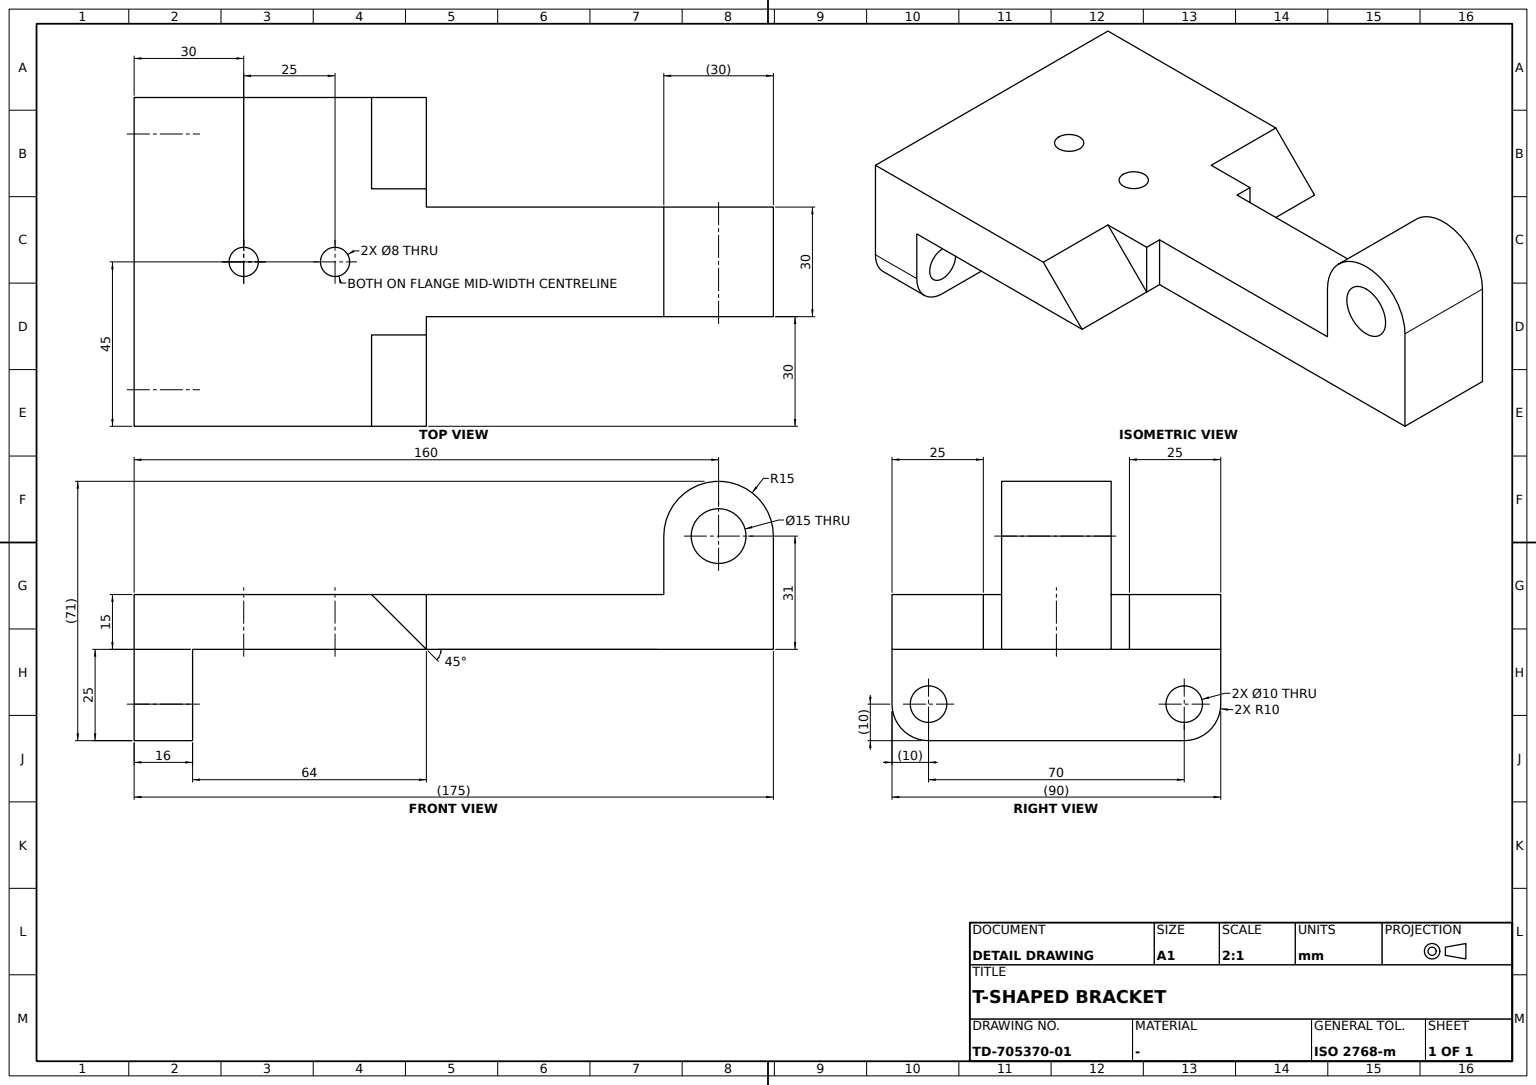
ISO-10303-21;
HEADER;
FILE_DESCRIPTION((''),'2;1');
FILE_NAME('','',(''),(''),'','','');
FILE_SCHEMA(('AUTOMOTIVE_DESIGN'));
ENDSEC;
DATA;
#1=APPLICATION_CONTEXT('');
#2=PRODUCT_CONTEXT('',#1,'mechanical');
#3=PRODUCT('','','',(#2));
#4=PRODUCT_DEFINITION_FORMATION('','',#3);
#5=PRODUCT_DEFINITION_CONTEXT('',#1,'design');
#6=PRODUCT_DEFINITION('','',#4,#5);
#7=PRODUCT_DEFINITION_SHAPE('','',#6);
#8=(LENGTH_UNIT()NAMED_UNIT(*)SI_UNIT(.MILLI.,.METRE.));
#9=(NAMED_UNIT(*)PLANE_ANGLE_UNIT()SI_UNIT($,.RADIAN.));
#10=(NAMED_UNIT(*)SI_UNIT($,.STERADIAN.)SOLID_ANGLE_UNIT());
#11=UNCERTAINTY_MEASURE_WITH_UNIT(LENGTH_MEASURE(0.005),#8,'distance_accuracy_value','');
#12=(GEOMETRIC_REPRESENTATION_CONTEXT(3)GLOBAL_UNCERTAINTY_ASSIGNED_CONTEXT((#11))GLOBAL_UNIT_ASSIGNED_CONTEXT((#8,#9,#10))REPRESENTATION_CONTEXT('',''));
#13=CARTESIAN_POINT('',(160.,-15.,38.5));
#14=VERTEX_POINT('',#13);
#15=CARTESIAN_POINT('',(160.,15.,38.5));
#16=VERTEX_POINT('',#15);
#17=CARTESIAN_POINT('',(160.,75.,38.5));
#18=DIRECTION('',(0.,-1.,0.));
#19=VECTOR('',#18,1000.);
#20=LINE('',#17,#19);
#21=EDGE_CURVE('',#14,#16,#20,.F.);
#22=ORIENTED_EDGE('',*,*,#21,.T.);
#23=CARTESIAN_POINT('',(160.,15.,23.5));
#24=VERTEX_POINT('',#23);
#25=CARTESIAN_POINT('',(160.,15.,31.));
#26=DIRECTION('',(0.,1.,0.));
#27=DIRECTION('',(0.,0.,1.));
#28=AXIS2_PLACEMENT_3D('',#25,#26,#27);
#29=CIRCLE('',#28,7.5);
#30=EDGE_CURVE('',#16,#24,#29,.T.);
#31=ORIENTED_EDGE('',*,*,#30,.T.);
#32=CARTESIAN_POINT('',(160.,-15.,23.5));
#33=VERTEX_POINT('',#32);
#34=CARTESIAN_POINT('',(160.,75.,23.5));
#35=LINE('',#34,#19);
#36=EDGE_CURVE('',#24,#33,#35,.T.);
#37=ORIENTED_EDGE('',*,*,#36,.T.);
#38=CARTESIAN_POINT('',(160.,-15.,31.));
#39=DIRECTION('',(1.,0.,0.));
#40=AXIS2_PLACEMENT_3D('',#38,#18,#39);
#41=CIRCLE('',#40,7.5);
#42=EDGE_CURVE('',#33,#14,#41,.T.);
#43=ORIENTED_EDGE('',*,*,#42,.T.);
#44=EDGE_LOOP('',(#22,#31,#37,#43));
#45=FACE_BOUND('',#44,.T.);
#46=CARTESIAN_POINT('',(160.,75.,31.));
#47=DIRECTION('',(0.,0.,-1.));
#48=AXIS2_PLACEMENT_3D('',#46,#18,#47);
#49=CYLINDRICAL_SURFACE('',#48,7.5);
#50=ADVANCED_FACE('',(#45),#49,.F.);
#51=CARTESIAN_POINT('',(0.,-35.,-10.));
#52=VERTEX_POINT('',#51);
#53=CARTESIAN_POINT('',(16.,-35.,-10.));
#54=VERTEX_POINT('',#53);
#55=DIRECTION('',(-1.,0.,0.));
#56=VECTOR('',#55,1000.);
#57=LINE('',#53,#56);
#58=EDGE_CURVE('',#52,#54,#57,.F.);
#59=ORIENTED_EDGE('',*,*,#58,.T.);
#60=CARTESIAN_POINT('',(16.,-35.,-20.));
#61=VERTEX_POINT('',#60);
#62=CARTESIAN_POINT('',(16.,-35.,-15.));
#63=AXIS2_PLACEMENT_3D('',#62,#39,#26);
#64=CIRCLE('',#63,5.);
#65=EDGE_CURVE('',#54,#61,#64,.T.);
#66=ORIENTED_EDGE('',*,*,#65,.T.);
#67=CARTESIAN_POINT('',(0.,-35.,-20.));
#68=VERTEX_POINT('',#67);
#69=LINE('',#60,#56);
#70=EDGE_CURVE('',#61,#68,#69,.T.);
#71=ORIENTED_EDGE('',*,*,#70,.T.);
#72=CARTESIAN_POINT('',(0.,-35.,-15.));
#73=AXIS2_PLACEMENT_3D('',#72,#39,#26);
#74=CIRCLE('',#73,5.);
#75=EDGE_CURVE('',#52,#68,#74,.T.);
#76=ORIENTED_EDGE('',*,*,#75,.F.);
#77=EDGE_LOOP('',(#59,#66,#71,#76));
#78=FACE_BOUND('',#77,.T.);
#79=AXIS2_PLACEMENT_3D('',#62,#55,#27);
#80=CYLINDRICAL_SURFACE('',#79,5.);
#81=ADVANCED_FACE('',(#78),#80,.F.);
#82=CARTESIAN_POINT('',(59.,0.,15.));
#83=VERTEX_POINT('',#82);
#84=CARTESIAN_POINT('',(51.,0.,15.));
#85=VERTEX_POINT('',#84);
#86=CARTESIAN_POINT('',(55.,0.,15.));
#87=AXIS2_PLACEMENT_3D('',#86,#27,#55);
#88=CIRCLE('',#87,4.);
#89=EDGE_CURVE('',#83,#85,#88,.T.);
#90=ORIENTED_EDGE('',*,*,#89,.T.);
#91=CARTESIAN_POINT('',(51.,0.,0.));
#92=VERTEX_POINT('',#91);
#93=CARTESIAN_POINT('',(51.,0.,90.));
#94=VECTOR('',#47,1000.);
#95=LINE('',#93,#94);
#96=EDGE_CURVE('',#85,#92,#95,.T.);
#97=ORIENTED_EDGE('',*,*,#96,.T.);
#98=CARTESIAN_POINT('',(59.,0.,0.));
#99=VERTEX_POINT('',#98);
#100=CARTESIAN_POINT('',(55.,0.,0.));
#101=AXIS2_PLACEMENT_3D('',#100,#27,#39);
#102=CIRCLE('',#101,4.);
#103=EDGE_CURVE('',#99,#92,#102,.T.);
#104=ORIENTED_EDGE('',*,*,#103,.F.);
#105=CARTESIAN_POINT('',(59.,0.,90.));
#106=LINE('',#105,#94);
#107=EDGE_CURVE('',#99,#83,#106,.F.);
#108=ORIENTED_EDGE('',*,*,#107,.T.);
#109=EDGE_LOOP('',(#90,#97,#104,#108));
#110=FACE_BOUND('',#109,.T.);
#111=CARTESIAN_POINT('',(55.,0.,90.));
#112=AXIS2_PLACEMENT_3D('',#111,#47,#55);
#113=CYLINDRICAL_SURFACE('',#112,4.);
#114=ADVANCED_FACE('',(#110),#113,.F.);
#115=CARTESIAN_POINT('',(0.,45.,15.));
#116=VERTEX_POINT('',#115);
#117=CARTESIAN_POINT('',(0.,45.,-15.));
#118=VERTEX_POINT('',#117);
#119=LINE('',#115,#94);
#120=EDGE_CURVE('',#116,#118,#119,.T.);
#121=ORIENTED_EDGE('',*,*,#120,.T.);
#122=CARTESIAN_POINT('',(0.,35.,-25.));
#123=VERTEX_POINT('',#122);
#124=CARTESIAN_POINT('',(0.,35.,-15.));
#125=AXIS2_PLACEMENT_3D('',#124,#55,#47);
#126=CIRCLE('',#125,10.);
#127=EDGE_CURVE('',#118,#123,#126,.T.);
#128=ORIENTED_EDGE('',*,*,#127,.T.);
#129=CARTESIAN_POINT('',(0.,-35.,-25.));
#130=VERTEX_POINT('',#129);
#131=CARTESIAN_POINT('',(0.,-45.,-25.));
#132=VECTOR('',#26,1000.);
#133=LINE('',#131,#132);
#134=EDGE_CURVE('',#130,#123,#133,.T.);
#135=ORIENTED_EDGE('',*,*,#134,.F.);
#136=CARTESIAN_POINT('',(0.,-45.,-15.));
#137=VERTEX_POINT('',#136);
#138=AXIS2_PLACEMENT_3D('',#72,#55,#47);
#139=CIRCLE('',#138,10.);
#140=EDGE_CURVE('',#130,#137,#139,.T.);
#141=ORIENTED_EDGE('',*,*,#140,.T.);
#142=CARTESIAN_POINT('',(0.,-45.,15.));
#143=VERTEX_POINT('',#142);
#144=LINE('',#142,#94);
#145=EDGE_CURVE('',#143,#137,#144,.T.);
#146=ORIENTED_EDGE('',*,*,#145,.F.);
#147=LINE('',#142,#132);
#148=EDGE_CURVE('',#143,#116,#147,.T.);
#149=ORIENTED_EDGE('',*,*,#148,.T.);
#150=EDGE_LOOP('',(#121,#128,#135,#141,#146,#149));
#151=FACE_BOUND('',#150,.T.);
#152=ORIENTED_EDGE('',*,*,#75,.T.);
#153=EDGE_CURVE('',#68,#52,#74,.T.);
#154=ORIENTED_EDGE('',*,*,#153,.T.);
#155=EDGE_LOOP('',(#152,#154));
#156=FACE_BOUND('',#155,.T.);
#157=CARTESIAN_POINT('',(0.,35.,-10.));
#158=VERTEX_POINT('',#157);
#159=CARTESIAN_POINT('',(0.,35.,-20.));
#160=VERTEX_POINT('',#159);
#161=AXIS2_PLACEMENT_3D('',#124,#39,#26);
#162=CIRCLE('',#161,5.);
#163=EDGE_CURVE('',#158,#160,#162,.T.);
#164=ORIENTED_EDGE('',*,*,#163,.T.);
#165=EDGE_CURVE('',#160,#158,#162,.T.);
#166=ORIENTED_EDGE('',*,*,#165,.T.);
#167=EDGE_LOOP('',(#164,#166));
#168=FACE_BOUND('',#167,.T.);
#169=AXIS2_PLACEMENT_3D('',#142,#39,#47);
#170=PLANE('',#169);
#171=ADVANCED_FACE('',(#151,#156,#168),#170,.F.);
#172=CARTESIAN_POINT('',(145.,-15.,31.));
#173=VERTEX_POINT('',#172);
#174=CARTESIAN_POINT('',(175.,-15.,31.));
#175=VERTEX_POINT('',#174);
#176=AXIS2_PLACEMENT_3D('',#38,#26,#39);
#177=CIRCLE('',#176,15.);
#178=EDGE_CURVE('',#173,#175,#177,.T.);
#179=ORIENTED_EDGE('',*,*,#178,.F.);
#180=CARTESIAN_POINT('',(145.,-15.,15.));
#181=VERTEX_POINT('',#180);
#182=CARTESIAN_POINT('',(145.,-15.,46.));
#183=LINE('',#182,#94);
#184=EDGE_CURVE('',#173,#181,#183,.T.);
#185=ORIENTED_EDGE('',*,*,#184,.T.);
#186=CARTESIAN_POINT('',(80.,-15.,15.));
#187=VERTEX_POINT('',#186);
#188=LINE('',#180,#56);
#189=EDGE_CURVE('',#181,#187,#188,.T.);
#190=ORIENTED_EDGE('',*,*,#189,.T.);
#191=CARTESIAN_POINT('',(80.,-15.,0.));
#192=VERTEX_POINT('',#191);
#193=CARTESIAN_POINT('',(80.,-15.,90.));
#194=VECTOR('',#27,1000.);
#195=LINE('',#193,#194);
#196=EDGE_CURVE('',#192,#187,#195,.T.);
#197=ORIENTED_EDGE('',*,*,#196,.F.);
#198=CARTESIAN_POINT('',(175.,-15.,0.));
#199=VERTEX_POINT('',#198);
#200=LINE('',#198,#56);
#201=EDGE_CURVE('',#199,#192,#200,.T.);
#202=ORIENTED_EDGE('',*,*,#201,.F.);
#203=CARTESIAN_POINT('',(175.,-15.,90.));
#204=LINE('',#203,#94);
#205=EDGE_CURVE('',#175,#199,#204,.T.);
#206=ORIENTED_EDGE('',*,*,#205,.F.);
#207=EDGE_LOOP('',(#179,#185,#190,#197,#202,#206));
#208=FACE_BOUND('',#207,.T.);
#209=ORIENTED_EDGE('',*,*,#42,.F.);
#210=EDGE_CURVE('',#14,#33,#41,.T.);
#211=ORIENTED_EDGE('',*,*,#210,.F.);
#212=EDGE_LOOP('',(#209,#211));
#213=FACE_BOUND('',#212,.T.);
#214=AXIS2_PLACEMENT_3D('',#203,#18,#47);
#215=PLANE('',#214);
#216=ADVANCED_FACE('',(#208,#213),#215,.T.);
#217=CARTESIAN_POINT('',(80.,20.,15.));
#218=VERTEX_POINT('',#217);
#219=CARTESIAN_POINT('',(80.,20.,0.));
#220=VERTEX_POINT('',#219);
#221=LINE('',#217,#94);
#222=EDGE_CURVE('',#218,#220,#221,.T.);
#223=ORIENTED_EDGE('',*,*,#222,.F.);
#224=CARTESIAN_POINT('',(80.,15.,15.));
#225=VERTEX_POINT('',#224);
#226=CARTESIAN_POINT('',(80.,-45.,15.));
#227=LINE('',#226,#19);
#228=EDGE_CURVE('',#218,#225,#227,.T.);
#229=ORIENTED_EDGE('',*,*,#228,.T.);
#230=CARTESIAN_POINT('',(80.,15.,0.));
#231=VERTEX_POINT('',#230);
#232=CARTESIAN_POINT('',(80.,15.,90.));
#233=LINE('',#232,#194);
#234=EDGE_CURVE('',#231,#225,#233,.T.);
#235=ORIENTED_EDGE('',*,*,#234,.F.);
#236=CARTESIAN_POINT('',(80.,45.,0.));
#237=LINE('',#236,#19);
#238=EDGE_CURVE('',#220,#231,#237,.T.);
#239=ORIENTED_EDGE('',*,*,#238,.F.);
#240=EDGE_LOOP('',(#223,#229,#235,#239));
#241=FACE_BOUND('',#240,.T.);
#242=CARTESIAN_POINT('',(80.,45.,90.));
#243=AXIS2_PLACEMENT_3D('',#242,#39,#47);
#244=PLANE('',#243);
#245=ADVANCED_FACE('',(#241),#244,.T.);
#246=ORIENTED_EDGE('',*,*,#70,.F.);
#247=EDGE_CURVE('',#61,#54,#64,.T.);
#248=ORIENTED_EDGE('',*,*,#247,.T.);
#249=ORIENTED_EDGE('',*,*,#58,.F.);
#250=ORIENTED_EDGE('',*,*,#153,.F.);
#251=EDGE_LOOP('',(#246,#248,#249,#250));
#252=FACE_BOUND('',#251,.T.);
#253=ADVANCED_FACE('',(#252),#80,.F.);
#254=ORIENTED_EDGE('',*,*,#247,.F.);
#255=ORIENTED_EDGE('',*,*,#65,.F.);
#256=EDGE_LOOP('',(#254,#255));
#257=FACE_BOUND('',#256,.T.);
#258=CARTESIAN_POINT('',(16.,-35.,-25.));
#259=VERTEX_POINT('',#258);
#260=CARTESIAN_POINT('',(16.,35.,-25.));
#261=VERTEX_POINT('',#260);
#262=CARTESIAN_POINT('',(16.,-45.,-25.));
#263=LINE('',#262,#132);
#264=EDGE_CURVE('',#259,#261,#263,.T.);
#265=ORIENTED_EDGE('',*,*,#264,.T.);
#266=CARTESIAN_POINT('',(16.,45.,-15.));
#267=VERTEX_POINT('',#266);
#268=CARTESIAN_POINT('',(16.,35.,-15.));
#269=AXIS2_PLACEMENT_3D('',#268,#39,#27);
#270=CIRCLE('',#269,10.);
#271=EDGE_CURVE('',#261,#267,#270,.T.);
#272=ORIENTED_EDGE('',*,*,#271,.T.);
#273=CARTESIAN_POINT('',(16.,45.,0.));
#274=VERTEX_POINT('',#273);
#275=CARTESIAN_POINT('',(16.,45.,-25.));
#276=LINE('',#275,#194);
#277=EDGE_CURVE('',#267,#274,#276,.T.);
#278=ORIENTED_EDGE('',*,*,#277,.T.);
#279=CARTESIAN_POINT('',(16.,-45.,0.));
#280=VERTEX_POINT('',#279);
#281=LINE('',#279,#132);
#282=EDGE_CURVE('',#280,#274,#281,.T.);
#283=ORIENTED_EDGE('',*,*,#282,.F.);
#284=CARTESIAN_POINT('',(16.,-45.,-15.));
#285=VERTEX_POINT('',#284);
#286=LINE('',#262,#194);
#287=EDGE_CURVE('',#285,#280,#286,.T.);
#288=ORIENTED_EDGE('',*,*,#287,.F.);
#289=AXIS2_PLACEMENT_3D('',#62,#39,#27);
#290=CIRCLE('',#289,10.);
#291=EDGE_CURVE('',#285,#259,#290,.T.);
#292=ORIENTED_EDGE('',*,*,#291,.T.);
#293=EDGE_LOOP('',(#265,#272,#278,#283,#288,#292));
#294=FACE_BOUND('',#293,.T.);
#295=CARTESIAN_POINT('',(16.,35.,-20.));
#296=VERTEX_POINT('',#295);
#297=CARTESIAN_POINT('',(16.,35.,-10.));
#298=VERTEX_POINT('',#297);
#299=AXIS2_PLACEMENT_3D('',#268,#39,#26);
#300=CIRCLE('',#299,5.);
#301=EDGE_CURVE('',#296,#298,#300,.T.);
#302=ORIENTED_EDGE('',*,*,#301,.F.);
#303=EDGE_CURVE('',#298,#296,#300,.T.);
#304=ORIENTED_EDGE('',*,*,#303,.F.);
#305=EDGE_LOOP('',(#302,#304));
#306=FACE_BOUND('',#305,.T.);
#307=AXIS2_PLACEMENT_3D('',#262,#55,#27);
#308=PLANE('',#307);
#309=ADVANCED_FACE('',(#257,#294,#306),#308,.F.);
#310=ORIENTED_EDGE('',*,*,#301,.T.);
#311=LINE('',#297,#56);
#312=EDGE_CURVE('',#158,#298,#311,.F.);
#313=ORIENTED_EDGE('',*,*,#312,.F.);
#314=ORIENTED_EDGE('',*,*,#165,.F.);
#315=LINE('',#295,#56);
#316=EDGE_CURVE('',#296,#160,#315,.T.);
#317=ORIENTED_EDGE('',*,*,#316,.F.);
#318=EDGE_LOOP('',(#310,#313,#314,#317));
#319=FACE_BOUND('',#318,.T.);
#320=AXIS2_PLACEMENT_3D('',#268,#55,#27);
#321=CYLINDRICAL_SURFACE('',#320,5.);
#322=ADVANCED_FACE('',(#319),#321,.F.);
#323=EDGE_CURVE('',#85,#83,#88,.T.);
#324=ORIENTED_EDGE('',*,*,#323,.F.);
#325=ORIENTED_EDGE('',*,*,#89,.F.);
#326=EDGE_LOOP('',(#324,#325));
#327=FACE_BOUND('',#326,.T.);
#328=CARTESIAN_POINT('',(34.,0.,15.));
#329=VERTEX_POINT('',#328);
#330=CARTESIAN_POINT('',(26.,0.,15.));
#331=VERTEX_POINT('',#330);
#332=CARTESIAN_POINT('',(30.,0.,15.));
#333=AXIS2_PLACEMENT_3D('',#332,#27,#55);
#334=CIRCLE('',#333,4.);
#335=EDGE_CURVE('',#329,#331,#334,.T.);
#336=ORIENTED_EDGE('',*,*,#335,.F.);
#337=EDGE_CURVE('',#331,#329,#334,.T.);
#338=ORIENTED_EDGE('',*,*,#337,.F.);
#339=EDGE_LOOP('',(#336,#338));
#340=FACE_BOUND('',#339,.T.);
#341=CARTESIAN_POINT('',(65.,45.,15.));
#342=VERTEX_POINT('',#341);
#343=CARTESIAN_POINT('',(65.,20.,15.));
#344=VERTEX_POINT('',#343);
#345=LINE('',#341,#19);
#346=EDGE_CURVE('',#342,#344,#345,.T.);
#347=ORIENTED_EDGE('',*,*,#346,.F.);
#348=CARTESIAN_POINT('',(145.,45.,15.));
#349=LINE('',#348,#56);
#350=EDGE_CURVE('',#342,#116,#349,.T.);
#351=ORIENTED_EDGE('',*,*,#350,.T.);
#352=ORIENTED_EDGE('',*,*,#148,.F.);
#353=CARTESIAN_POINT('',(65.,-45.,15.));
#354=VERTEX_POINT('',#353);
#355=CARTESIAN_POINT('',(145.,-45.,15.));
#356=LINE('',#355,#56);
#357=EDGE_CURVE('',#354,#143,#356,.T.);
#358=ORIENTED_EDGE('',*,*,#357,.F.);
#359=CARTESIAN_POINT('',(65.,-20.,15.));
#360=VERTEX_POINT('',#359);
#361=LINE('',#353,#132);
#362=EDGE_CURVE('',#354,#360,#361,.T.);
#363=ORIENTED_EDGE('',*,*,#362,.T.);
#364=CARTESIAN_POINT('',(80.,-20.,15.));
#365=VERTEX_POINT('',#364);
#366=LINE('',#364,#56);
#367=EDGE_CURVE('',#365,#360,#366,.T.);
#368=ORIENTED_EDGE('',*,*,#367,.F.);
#369=EDGE_CURVE('',#187,#365,#227,.T.);
#370=ORIENTED_EDGE('',*,*,#369,.F.);
#371=ORIENTED_EDGE('',*,*,#189,.F.);
#372=CARTESIAN_POINT('',(145.,15.,15.));
#373=VERTEX_POINT('',#372);
#374=LINE('',#355,#132);
#375=EDGE_CURVE('',#181,#373,#374,.T.);
#376=ORIENTED_EDGE('',*,*,#375,.T.);
#377=VECTOR('',#39,1000.);
#378=LINE('',#372,#377);
#379=EDGE_CURVE('',#225,#373,#378,.T.);
#380=ORIENTED_EDGE('',*,*,#379,.F.);
#381=ORIENTED_EDGE('',*,*,#228,.F.);
#382=LINE('',#343,#377);
#383=EDGE_CURVE('',#344,#218,#382,.T.);
#384=ORIENTED_EDGE('',*,*,#383,.F.);
#385=EDGE_LOOP('',(#347,#351,#352,#358,#363,#368,#370,#371,#376,#380,#381,#384));
#386=FACE_BOUND('',#385,.T.);
#387=AXIS2_PLACEMENT_3D('',#355,#47,#55);
#388=PLANE('',#387);
#389=ADVANCED_FACE('',(#327,#340,#386),#388,.F.);
#390=CARTESIAN_POINT('',(145.,15.,31.));
#391=VERTEX_POINT('',#390);
#392=CARTESIAN_POINT('',(145.,75.,31.));
#393=LINE('',#392,#19);
#394=EDGE_CURVE('',#391,#173,#393,.T.);
#395=ORIENTED_EDGE('',*,*,#394,.F.);
#396=CARTESIAN_POINT('',(145.,15.,46.));
#397=LINE('',#396,#194);
#398=EDGE_CURVE('',#373,#391,#397,.T.);
#399=ORIENTED_EDGE('',*,*,#398,.F.);
#400=ORIENTED_EDGE('',*,*,#375,.F.);
#401=ORIENTED_EDGE('',*,*,#184,.F.);
#402=EDGE_LOOP('',(#395,#399,#400,#401));
#403=FACE_BOUND('',#402,.T.);
#404=CARTESIAN_POINT('',(145.,-45.,46.));
#405=AXIS2_PLACEMENT_3D('',#404,#39,#47);
#406=PLANE('',#405);
#407=ADVANCED_FACE('',(#403),#406,.F.);
#408=ORIENTED_EDGE('',*,*,#316,.T.);
#409=ORIENTED_EDGE('',*,*,#163,.F.);
#410=ORIENTED_EDGE('',*,*,#312,.T.);
#411=ORIENTED_EDGE('',*,*,#303,.T.);
#412=EDGE_LOOP('',(#408,#409,#410,#411));
#413=FACE_BOUND('',#412,.T.);
#414=ADVANCED_FACE('',(#413),#321,.F.);
#415=CARTESIAN_POINT('',(175.,15.,31.));
#416=VERTEX_POINT('',#415);
#417=CARTESIAN_POINT('',(175.,75.,31.));
#418=LINE('',#417,#19);
#419=EDGE_CURVE('',#416,#175,#418,.T.);
#420=ORIENTED_EDGE('',*,*,#419,.T.);
#421=ORIENTED_EDGE('',*,*,#205,.T.);
#422=CARTESIAN_POINT('',(175.,15.,0.));
#423=VERTEX_POINT('',#422);
#424=CARTESIAN_POINT('',(175.,-45.,0.));
#425=LINE('',#424,#132);
#426=EDGE_CURVE('',#199,#423,#425,.T.);
#427=ORIENTED_EDGE('',*,*,#426,.T.);
#428=CARTESIAN_POINT('',(175.,15.,90.));
#429=LINE('',#428,#94);
#430=EDGE_CURVE('',#416,#423,#429,.T.);
#431=ORIENTED_EDGE('',*,*,#430,.F.);
#432=EDGE_LOOP('',(#420,#421,#427,#431));
#433=FACE_BOUND('',#432,.T.);
#434=AXIS2_PLACEMENT_3D('',#424,#55,#27);
#435=PLANE('',#434);
#436=ADVANCED_FACE('',(#433),#435,.F.);
#437=ORIENTED_EDGE('',*,*,#398,.T.);
#438=AXIS2_PLACEMENT_3D('',#25,#18,#27);
#439=CIRCLE('',#438,15.);
#440=EDGE_CURVE('',#416,#391,#439,.T.);
#441=ORIENTED_EDGE('',*,*,#440,.F.);
#442=ORIENTED_EDGE('',*,*,#430,.T.);
#443=LINE('',#230,#377);
#444=EDGE_CURVE('',#231,#423,#443,.T.);
#445=ORIENTED_EDGE('',*,*,#444,.F.);
#446=ORIENTED_EDGE('',*,*,#234,.T.);
#447=ORIENTED_EDGE('',*,*,#379,.T.);
#448=EDGE_LOOP('',(#437,#441,#442,#445,#446,#447));
#449=FACE_BOUND('',#448,.T.);
#450=EDGE_CURVE('',#24,#16,#29,.T.);
#451=ORIENTED_EDGE('',*,*,#450,.F.);
#452=ORIENTED_EDGE('',*,*,#30,.F.);
#453=EDGE_LOOP('',(#451,#452));
#454=FACE_BOUND('',#453,.T.);
#455=AXIS2_PLACEMENT_3D('',#232,#26,#27);
#456=PLANE('',#455);
#457=ADVANCED_FACE('',(#449,#454),#456,.T.);
#458=ORIENTED_EDGE('',*,*,#383,.T.);
#459=ORIENTED_EDGE('',*,*,#222,.T.);
#460=DIRECTION('',(-0.707106781,0.,0.707106781));
#461=VECTOR('',#460,1000.);
#462=LINE('',#219,#461);
#463=EDGE_CURVE('',#220,#344,#462,.T.);
#464=ORIENTED_EDGE('',*,*,#463,.T.);
#465=EDGE_LOOP('',(#458,#459,#464));
#466=FACE_BOUND('',#465,.T.);
#467=CARTESIAN_POINT('',(0.,20.,0.));
#468=AXIS2_PLACEMENT_3D('',#467,#26,#27);
#469=PLANE('',#468);
#470=ADVANCED_FACE('',(#466),#469,.T.);
#471=CARTESIAN_POINT('',(80.,-45.,0.));
#472=VERTEX_POINT('',#471);
#473=DIRECTION('',(0.707106781,0.,-0.707106781));
#474=VECTOR('',#473,1000.);
#475=LINE('',#353,#474);
#476=EDGE_CURVE('',#354,#472,#475,.T.);
#477=ORIENTED_EDGE('',*,*,#476,.T.);
#478=CARTESIAN_POINT('',(80.,-20.,0.));
#479=VERTEX_POINT('',#478);
#480=LINE('',#471,#132);
#481=EDGE_CURVE('',#472,#479,#480,.T.);
#482=ORIENTED_EDGE('',*,*,#481,.T.);
#483=LINE('',#359,#461);
#484=EDGE_CURVE('',#479,#360,#483,.T.);
#485=ORIENTED_EDGE('',*,*,#484,.T.);
#486=ORIENTED_EDGE('',*,*,#362,.F.);
#487=EDGE_LOOP('',(#477,#482,#485,#486));
#488=FACE_BOUND('',#487,.T.);
#489=DIRECTION('',(0.707106781,0.,0.707106781));
#490=AXIS2_PLACEMENT_3D('',#353,#489,#473);
#491=PLANE('',#490);
#492=ADVANCED_FACE('',(#488),#491,.T.);
#493=ORIENTED_EDGE('',*,*,#196,.T.);
#494=ORIENTED_EDGE('',*,*,#369,.T.);
#495=LINE('',#478,#194);
#496=EDGE_CURVE('',#479,#365,#495,.T.);
#497=ORIENTED_EDGE('',*,*,#496,.F.);
#498=LINE('',#191,#19);
#499=EDGE_CURVE('',#192,#479,#498,.T.);
#500=ORIENTED_EDGE('',*,*,#499,.F.);
#501=EDGE_LOOP('',(#493,#494,#497,#500));
#502=FACE_BOUND('',#501,.T.);
#503=AXIS2_PLACEMENT_3D('',#193,#39,#47);
#504=PLANE('',#503);
#505=ADVANCED_FACE('',(#502),#504,.T.);
#506=ORIENTED_EDGE('',*,*,#36,.F.);
#507=ORIENTED_EDGE('',*,*,#450,.T.);
#508=ORIENTED_EDGE('',*,*,#21,.F.);
#509=ORIENTED_EDGE('',*,*,#210,.T.);
#510=EDGE_LOOP('',(#506,#507,#508,#509));
#511=FACE_BOUND('',#510,.T.);
#512=ADVANCED_FACE('',(#511),#49,.F.);
#513=ORIENTED_EDGE('',*,*,#367,.T.);
#514=ORIENTED_EDGE('',*,*,#484,.F.);
#515=ORIENTED_EDGE('',*,*,#496,.T.);
#516=EDGE_LOOP('',(#513,#514,#515));
#517=FACE_BOUND('',#516,.T.);
#518=CARTESIAN_POINT('',(0.,-20.,0.));
#519=AXIS2_PLACEMENT_3D('',#518,#18,#47);
#520=PLANE('',#519);
#521=ADVANCED_FACE('',(#517),#520,.T.);
#522=CARTESIAN_POINT('',(34.,0.,0.));
#523=VERTEX_POINT('',#522);
#524=CARTESIAN_POINT('',(34.,0.,90.));
#525=LINE('',#524,#94);
#526=EDGE_CURVE('',#329,#523,#525,.T.);
#527=ORIENTED_EDGE('',*,*,#526,.T.);
#528=CARTESIAN_POINT('',(26.,0.,0.));
#529=VERTEX_POINT('',#528);
#530=CARTESIAN_POINT('',(30.,0.,0.));
#531=AXIS2_PLACEMENT_3D('',#530,#27,#39);
#532=CIRCLE('',#531,4.);
#533=EDGE_CURVE('',#529,#523,#532,.T.);
#534=ORIENTED_EDGE('',*,*,#533,.F.);
#535=CARTESIAN_POINT('',(26.,0.,90.));
#536=LINE('',#535,#94);
#537=EDGE_CURVE('',#529,#331,#536,.F.);
#538=ORIENTED_EDGE('',*,*,#537,.T.);
#539=ORIENTED_EDGE('',*,*,#337,.T.);
#540=EDGE_LOOP('',(#527,#534,#538,#539));
#541=FACE_BOUND('',#540,.T.);
#542=CARTESIAN_POINT('',(30.,0.,90.));
#543=AXIS2_PLACEMENT_3D('',#542,#47,#55);
#544=CYLINDRICAL_SURFACE('',#543,4.);
#545=ADVANCED_FACE('',(#541),#544,.F.);
#546=ORIENTED_EDGE('',*,*,#271,.F.);
#547=LINE('',#122,#377);
#548=EDGE_CURVE('',#123,#261,#547,.T.);
#549=ORIENTED_EDGE('',*,*,#548,.F.);
#550=ORIENTED_EDGE('',*,*,#127,.F.);
#551=LINE('',#117,#56);
#552=EDGE_CURVE('',#267,#118,#551,.T.);
#553=ORIENTED_EDGE('',*,*,#552,.F.);
#554=EDGE_LOOP('',(#546,#549,#550,#553));
#555=FACE_BOUND('',#554,.T.);
#556=AXIS2_PLACEMENT_3D('',#124,#39,#47);
#557=CYLINDRICAL_SURFACE('',#556,10.);
#558=ADVANCED_FACE('',(#555),#557,.T.);
#559=ORIENTED_EDGE('',*,*,#96,.F.);
#560=ORIENTED_EDGE('',*,*,#323,.T.);
#561=ORIENTED_EDGE('',*,*,#107,.F.);
#562=EDGE_CURVE('',#92,#99,#102,.T.);
#563=ORIENTED_EDGE('',*,*,#562,.F.);
#564=EDGE_LOOP('',(#559,#560,#561,#563));
#565=FACE_BOUND('',#564,.T.);
#566=ADVANCED_FACE('',(#565),#113,.F.);
#567=EDGE_CURVE('',#523,#529,#532,.T.);
#568=ORIENTED_EDGE('',*,*,#567,.F.);
#569=ORIENTED_EDGE('',*,*,#526,.F.);
#570=ORIENTED_EDGE('',*,*,#335,.T.);
#571=ORIENTED_EDGE('',*,*,#537,.F.);
#572=EDGE_LOOP('',(#568,#569,#570,#571));
#573=FACE_BOUND('',#572,.T.);
#574=ADVANCED_FACE('',(#573),#544,.F.);
#575=ORIENTED_EDGE('',*,*,#357,.T.);
#576=ORIENTED_EDGE('',*,*,#145,.T.);
#577=LINE('',#284,#377);
#578=EDGE_CURVE('',#137,#285,#577,.T.);
#579=ORIENTED_EDGE('',*,*,#578,.T.);
#580=ORIENTED_EDGE('',*,*,#287,.T.);
#581=LINE('',#279,#377);
#582=EDGE_CURVE('',#280,#472,#581,.T.);
#583=ORIENTED_EDGE('',*,*,#582,.T.);
#584=ORIENTED_EDGE('',*,*,#476,.F.);
#585=EDGE_LOOP('',(#575,#576,#579,#580,#583,#584));
#586=FACE_BOUND('',#585,.T.);
#587=CARTESIAN_POINT('',(0.,-45.,0.));
#588=AXIS2_PLACEMENT_3D('',#587,#18,#47);
#589=PLANE('',#588);
#590=ADVANCED_FACE('',(#586),#589,.T.);
#591=VERTEX_POINT('',#236);
#592=LINE('',#273,#377);
#593=EDGE_CURVE('',#274,#591,#592,.T.);
#594=ORIENTED_EDGE('',*,*,#593,.F.);
#595=ORIENTED_EDGE('',*,*,#277,.F.);
#596=ORIENTED_EDGE('',*,*,#552,.T.);
#597=ORIENTED_EDGE('',*,*,#120,.F.);
#598=ORIENTED_EDGE('',*,*,#350,.F.);
#599=LINE('',#236,#461);
#600=EDGE_CURVE('',#591,#342,#599,.T.);
#601=ORIENTED_EDGE('',*,*,#600,.F.);
#602=EDGE_LOOP('',(#594,#595,#596,#597,#598,#601));
#603=FACE_BOUND('',#602,.T.);
#604=CARTESIAN_POINT('',(0.,45.,0.));
#605=AXIS2_PLACEMENT_3D('',#604,#18,#47);
#606=PLANE('',#605);
#607=ADVANCED_FACE('',(#603),#606,.F.);
#608=LINE('',#129,#56);
#609=EDGE_CURVE('',#259,#130,#608,.T.);
#610=ORIENTED_EDGE('',*,*,#609,.F.);
#611=ORIENTED_EDGE('',*,*,#291,.F.);
#612=ORIENTED_EDGE('',*,*,#578,.F.);
#613=ORIENTED_EDGE('',*,*,#140,.F.);
#614=EDGE_LOOP('',(#610,#611,#612,#613));
#615=FACE_BOUND('',#614,.T.);
#616=AXIS2_PLACEMENT_3D('',#72,#55,#27);
#617=CYLINDRICAL_SURFACE('',#616,10.);
#618=ADVANCED_FACE('',(#615),#617,.T.);
#619=ORIENTED_EDGE('',*,*,#419,.F.);
#620=ORIENTED_EDGE('',*,*,#440,.T.);
#621=ORIENTED_EDGE('',*,*,#394,.T.);
#622=ORIENTED_EDGE('',*,*,#178,.T.);
#623=EDGE_LOOP('',(#619,#620,#621,#622));
#624=FACE_BOUND('',#623,.T.);
#625=CYLINDRICAL_SURFACE('',#48,15.);
#626=ADVANCED_FACE('',(#624),#625,.T.);
#627=ORIENTED_EDGE('',*,*,#463,.F.);
#628=EDGE_CURVE('',#591,#220,#237,.T.);
#629=ORIENTED_EDGE('',*,*,#628,.F.);
#630=ORIENTED_EDGE('',*,*,#600,.T.);
#631=ORIENTED_EDGE('',*,*,#346,.T.);
#632=EDGE_LOOP('',(#627,#629,#630,#631));
#633=FACE_BOUND('',#632,.T.);
#634=AXIS2_PLACEMENT_3D('',#236,#489,#473);
#635=PLANE('',#634);
#636=ADVANCED_FACE('',(#633),#635,.T.);
#637=ORIENTED_EDGE('',*,*,#103,.T.);
#638=ORIENTED_EDGE('',*,*,#562,.T.);
#639=EDGE_LOOP('',(#637,#638));
#640=FACE_BOUND('',#639,.T.);
#641=ORIENTED_EDGE('',*,*,#567,.T.);
#642=ORIENTED_EDGE('',*,*,#533,.T.);
#643=EDGE_LOOP('',(#641,#642));
#644=FACE_BOUND('',#643,.T.);
#645=ORIENTED_EDGE('',*,*,#481,.F.);
#646=ORIENTED_EDGE('',*,*,#582,.F.);
#647=ORIENTED_EDGE('',*,*,#282,.T.);
#648=ORIENTED_EDGE('',*,*,#593,.T.);
#649=ORIENTED_EDGE('',*,*,#628,.T.);
#650=ORIENTED_EDGE('',*,*,#238,.T.);
#651=ORIENTED_EDGE('',*,*,#444,.T.);
#652=ORIENTED_EDGE('',*,*,#426,.F.);
#653=ORIENTED_EDGE('',*,*,#201,.T.);
#654=ORIENTED_EDGE('',*,*,#499,.T.);
#655=EDGE_LOOP('',(#645,#646,#647,#648,#649,#650,#651,#652,#653,#654));
#656=FACE_BOUND('',#655,.T.);
#657=AXIS2_PLACEMENT_3D('',#279,#27,#39);
#658=PLANE('',#657);
#659=ADVANCED_FACE('',(#640,#644,#656),#658,.F.);
#660=ORIENTED_EDGE('',*,*,#264,.F.);
#661=ORIENTED_EDGE('',*,*,#609,.T.);
#662=ORIENTED_EDGE('',*,*,#134,.T.);
#663=ORIENTED_EDGE('',*,*,#548,.T.);
#664=EDGE_LOOP('',(#660,#661,#662,#663));
#665=FACE_BOUND('',#664,.T.);
#666=AXIS2_PLACEMENT_3D('',#131,#27,#39);
#667=PLANE('',#666);
#668=ADVANCED_FACE('',(#665),#667,.F.);
#669=CLOSED_SHELL('',(#50,#81,#114,#171,#216,#245,#253,#309,#322,#389,#407,#414,#436,#457,#470,#492,#505,#512,#521,#545,#558,#566,#574,#590,#607,#618,#626,#636,#659,#668));
#670=MANIFOLD_SOLID_BREP('',#669);
#671=ADVANCED_BREP_SHAPE_REPRESENTATION('',(#670),#12);
#672=SHAPE_DEFINITION_REPRESENTATION(#7,#671);
ENDSEC;
END-ISO-10303-21;
